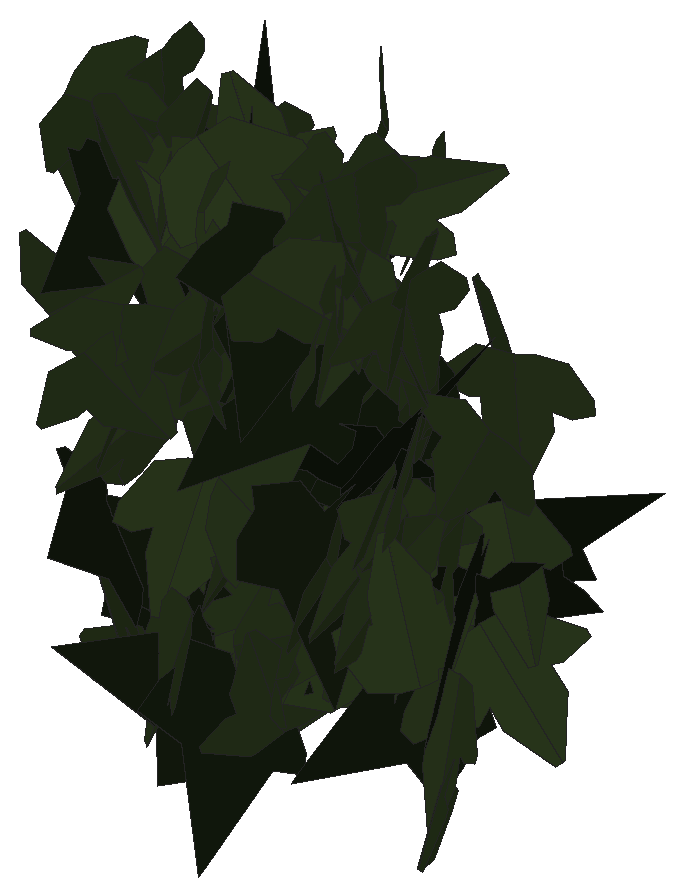
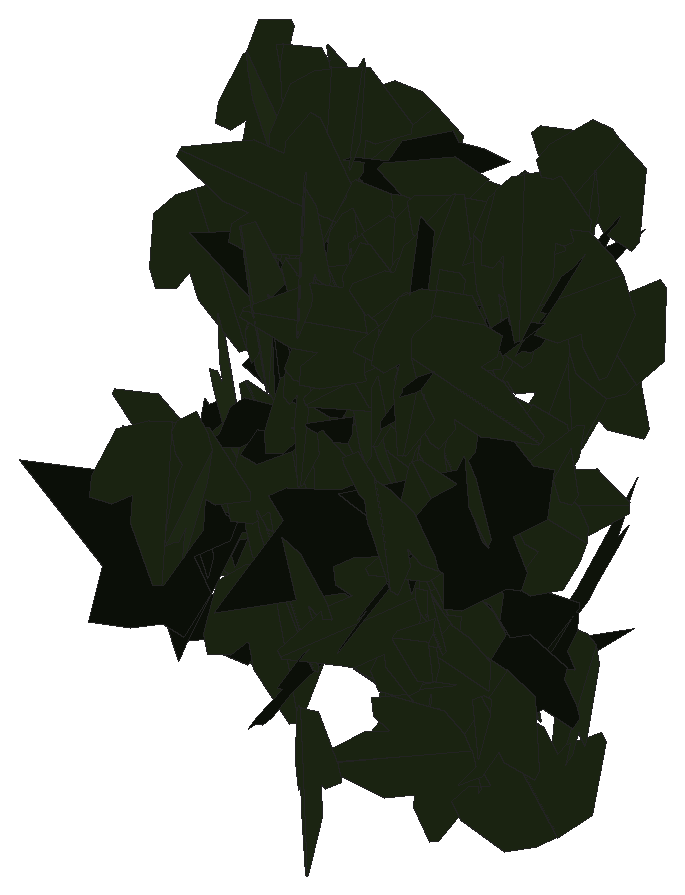
# SketchUp Ruby script. Lengths in inches.
U = 1.inch
M = Sketchup.active_model
def pt(a) = Geom::Point3d.new(a.map { |v| v * U })
def face(e, loops, mat)
  f = e.add_face(loops[0].map { |a| pt(a) })
  loops[1..].each { |l| e.add_face(l.map { |a| pt(a) }).erase! }
  f.material = f.back_material = mat if mat
  f
end
# faces: each face lists its corners as indices into pts; further lists are holes
def faces(e, pts, list, mat = nil) = list.each { |f| face(e, (f[0].is_a?(Array) ? f : [f]).map { |l| l.map { |i| pts[i] } }, mat) }
# xy, xz, yz: faces in a plane at the given z, y or x. An outline is a flat list of corners, or four numbers for a rectangle; further outlines are holes
def ring(l) = l.size == 4 ? [[l[0], l[1]], [l[2], l[1]], [l[2], l[3]], [l[0], l[3]]] : l.each_slice(2).to_a
def flat(e, list, mat, &to3) = list.each { |f| face(e, (f[0].is_a?(Array) ? f : [f]).map { |l| ring(l).map { |u, v| to3.(u, v) } }, mat) }
def xy(e, z, list, mat = nil) = flat(e, list, mat) { |x, y| [x, y, z] }
def xz(e, y, list, mat = nil) = flat(e, list, mat) { |x, z| [x, y, z] }
def yz(e, x, list, mat = nil) = flat(e, list, mat) { |y, z| [x, y, z] }
def lines(e, pts, list) = list.each { |a, b| e.add_line(pt(pts[a]), pt(pts[b])) }
# prism: a flat outline (further loops are holes) pulled along v
def prism(e, loops, v, mat = nil)
  f = face(e, loops, mat); d = Geom::Vector3d.new(v.map { |x| x * U })
  f.pushpull(f.normal.samedirection?(d) ? d.length : -d.length)
end
def box(e, o, s, mat = nil) = prism(e, [[o, [o[0] + s[0], o[1], o[2]], [o[0] + s[0], o[1] + s[1], o[2]], [o[0], o[1] + s[1], o[2]]]], [0, 0, s[2]], mat)
def at(x, y, z, deg = 0) = Geom::Transformation.translation(pt([x, y, z])) * Geom::Transformation.rotation(ORIGIN, Z_AXIS, deg.degrees)
def axes(o, x, y, z) = Geom::Transformation.new([*x, 0, *y, 0, *z, 0, *pt(o).to_a, 1])
def part(name) = M.definitions.add(name)
# library, detail: a bought-in or finely detailed component or shape, given as its bounding box
def library(name, o, s) = part(name).tap { |d| box(d.entities, o, s) }
def detail(e, o, s) = box(e.add_group.entities, o, s)
def put(e, d, t, mat = nil) = e.add_instance(d, t).tap { |i| i.material = mat if mat }
def group(e, t, mat = nil) = e.add_group.tap { |g| g.transformation = t; g.material = mat if mat }.entities
root = M.entities
M.materials.add("efeu1").color = [18, 25, 13]
M.materials.add("efeu2").color = [43, 57, 29]
c1 = part("ivyleaf_10")
p = [[0,0.5,-0.03],[-0.0625,2.02,-0.43],[-0.19,2.01,-0.46],[-0.54,1.05,-0.29],[-0.52,0.625,-0.18],[-0.83,0.76,-0.28],
  [-1.16,0.64,-0.33],[-1.15,0.33,-0.24],[-0.77,-0.39,0.02],[-0.3,-0.51,0.16],[0.04,-0.48,0.23],[-0.02,2.01,-0.4375],
  [-0.06,2.01,-0.43],[0.04,-0.49,0.23],[0.67,-0.49,0.14],[1.38,0.36,-0.2],[1.375,0.51,-0.24],[0.81,0.65,-0.19],
  [0.62,0.59,-0.15],[0.6,1.09,-0.28],[0.5,1.23,-0.31]]
faces(c1.entities,p,[[0,1,2,3,4,5,6,7,8,9,10],[11,12,0,13,14,15,16,17,18,19,20]],"efeu2")
c2 = part("ivyleaf_9")
p = [[1.54,2.16,1.25],[1.36,2.04,1.19],[-0.21,0.99,0.68],[-0.71,1.11,0.82],[-0.85,0.86,0.67],[-0.8,0.17,0.21],
  [-0.9,-0.01,0.1],[-0.67,-0.16,-0.02],[-0.08,-0.08,-0.05],[-0.03,-0.6,-0.4],[0.65,-0.88,-0.66],[0.83,-0.6,-0.49],
  [1.29,-0.42,-0.43],[1.8125,-0.07,-0.26],[1.21,0.44,0.15]]
faces(c2.entities,p,[[0,1,2,3,4,5,6,7,8,9,10,11,12,13,14]],"efeu1")
put(root,c1,axes([24.57,223.95,205.69],[-0.11682,0.10637,0.47438],[-0.34487,0.32575,-0.15797],[-0.34266,-0.36411,-0.00274]))
put(root,c1,axes([23.95,224.3125,202.88],[0.35736,-0.34773,-0.03714],[-0.02514,0.02743,-0.49861],[0.3488,0.35823,0.00212]))
put(root,c1,axes([25.12,224.07,206.5],[-0.27318,-0.1919,-0.37222],[0.30479,0.21365,-0.33385],[0.28718,-0.4093,0.00025]))
put(root,c1,axes([23.4375,224.29,205.45],[-0.40279,-0.29062,0.05747],[-0.04187,-0.04018,-0.49662],[0.29327,-0.40488,0.00803]))
put(root,c1,axes([22.87,224.29,205.4],[-0.33422,-0.06379,0.36637],[0.3582,0.07713,0.34021],[-0.09992,0.48988,-0.00586]))
put(root,c2,axes([24.93,224.52,206.46],[-0.27049,-0.41591,-0.06209],[0.03285,0.0527,-0.49613],[0.41924,-0.27247,-0.00118]))
put(root,c1,axes([24.61,224.3125,204.91],[-0.15567,-0.45543,0.13548],[0.0701,0.11899,0.48055],[-0.46995,0.16861,0.0268]))
put(root,c1,axes([26.24,224.26,206.63],[-0.18585,-0.43965,-0.14887],[0.05349,0.13901,-0.4773],[0.46108,-0.19334,-0.00464]))
put(root,c1,axes([24.77,224.08,204.48],[-0.00219,0.40153,0.29795],[-0.00192,0.29794,-0.40153],[-0.49999,-0.00291,0.00024]))
put(root,c2,axes([24.3125,224.65,202.32],[-0.11639,-0.48302,0.05608],[-0.01336,-0.05447,-0.49684],[0.48608,-0.11716,-0.00023]))
put(root,c1,axes([25.625,224.72,203.66],[-0.036,-0.03934,0.49715],[0.25855,-0.4277,-0.01512],[0.42645,0.25598,0.05114]))
put(root,c1,axes([23.3,224.2,205.09],[-0.28336,-0.30808,-0.27349],[0.17718,0.20853,-0.41848],[0.3719,-0.33407,-0.009]))
put(root,c1,axes([26.16,224.57,206.83],[0.22591,-0.4016,0.19412],[0.09855,-0.16728,-0.46077],[0.43503,0.24644,0.00357]))
put(root,c1,axes([25.63,224.75,204.15],[0.04581,-0.2235,0.44492],[0.10899,-0.43146,-0.22796],[0.48582,0.11787,0.00919]))
put(root,c2,axes([25.01,224.73,205.46],[-0.34584,-0.30956,0.18592],[-0.13083,-0.13252,-0.46403],[0.33657,-0.36961,0.01066]))
put(root,c2,axes([22.92,224.77,203.37],[0.28209,-0.27912,-0.30416],[0.21889,-0.21121,0.39684],[-0.35001,-0.35705,0.00303]))
put(root,c1,axes([25.25,224.63,206.56],[-0.15262,0.08956,0.46764],[0.41437,-0.2169,0.17678],[0.23452,0.44151,-0.00802]))
put(root,c1,axes([24.69,224.67,202.29],[-0.21464,-0.40409,-0.20159],[-0.08658,-0.18223,0.45749],[-0.44321,0.2313,0.00825]))
put(root,c2,axes([25.17,224.6,204.21],[-0.09776,-0.46401,-0.15855],[0.01898,0.15796,-0.47401],[0.48998,-0.0987,-0.01327]))
put(root,c1,axes([25.12,224.45,205.63],[0.27714,-0.41403,0.04202],[-0.01725,0.03901,0.49818],[-0.4158,-0.27758,0.00734]))
put(root,c1,axes([23.09,224.57,206.94],[-0.31088,0.21856,-0.32494],[0.25942,-0.19584,-0.37993],[-0.29334,-0.40482,0.00837]))
put(root,c2,axes([24.11,224.79,202.22],[-0.14487,-0.39163,-0.27502],[-0.0876,-0.26079,0.41751],[-0.47047,0.16915,0.00694]))
put(root,c1,axes([26.43,224.375,201.96],[0.27052,-0.35966,0.21786],[-0.13103,0.17405,0.45004],[-0.39956,-0.30058,-0.00009]))
put(root,c1,axes([24.4,224.87,204],[0.09608,-0.24805,0.42337],[0.1342,-0.40167,-0.2658],[0.47197,0.16471,-0.01061]))
put(root,c2,axes([23.03,224.95,206.03],[-0.10925,-0.28685,0.39469],[-0.09083,-0.38544,-0.30527],[0.47939,-0.1384,0.03211]))
put(root,c1,axes([26.33,224.68,202.94],[0.44053,-0.21342,0.10192],[0.09307,-0.04166,-0.48949],[0.21743,0.45024,0.00302]))
put(root,c1,axes([24.34,224.77,202.78],[0.1958,-0.1455,-0.43645],[0.33546,-0.27946,0.24366],[-0.31485,-0.38824,-0.01182]))
put(root,c1,axes([23.78,224.93,205.3],[-0.07333,0.08624,0.48702],[0.21879,-0.43589,0.11013],[0.44357,0.22926,0.0262]))
put(root,c1,axes([25.38,224.8,206.3],[0.01961,0.37311,-0.33227],[-0.03623,-0.33059,-0.37336],[-0.4983,0.03872,0.01407]))
put(root,c1,axes([25.32,224.45,203.92],[0.03509,-0.38631,-0.31549],[-0.01346,0.31542,-0.38772],[0.49859,0.0357,0.01173]))
put(root,c1,axes([23.12,225.03,204.28],[-0.01076,-0.14686,0.47782],[0.03165,-0.47718,-0.14595],[0.49888,0.02711,0.01957]))
put(root,c2,axes([25.77,224.34,204.92],[-0.07485,0.4794,-0.12073],[-0.03727,0.11628,0.48486],[0.49296,0.08159,0.01833]))
put(root,c1,axes([26,224.5625,205.76],[-0.29498,0.22202,-0.33719],[-0.2983,0.16153,0.36732],[0.27203,0.41787,0.03716]))
put(root,c1,axes([26.7,224.66,205.375],[-0.41664,-0.04093,0.27338],[-0.26963,-0.04881,-0.41823],[0.06093,-0.49593,0.0186]))
put(root,c1,axes([25.96,224.66,203.27],[0.16451,0.4717,0.02086],[-0.00695,-0.01967,0.49956],[0.47211,-0.16465,0.00008]))
put(root,c1,axes([25.77,224.78,204.51],[0.23603,-0.43595,-0.06509],[0.0358,-0.05463,0.49572],[-0.43933,-0.23867,0.00543]))
put(root,c1,axes([25.57,224.8,204.45],[0.25687,-0.42892,0.00667],[0.00341,-0.00573,-0.49996],[0.42896,0.25689,-0.00002]))
put(root,c1,axes([24.68,224.78,206.21],[0.48269,0.12391,0.04076],[0.03961,0.00966,-0.49834],[-0.12428,0.48431,-0.00049]))
put(root,c2,axes([25.87,225.16,202.75],[0.0077,-0.14569,-0.47824],[0.10224,-0.46773,0.14413],[-0.48938,-0.10001,0.02259]))
put(root,c1,axes([25.37,224.79,203.07],[0.34007,-0.01893,-0.36605],[-0.36326,0.04927,-0.34002],[0.04894,0.49721,0.01976]))
put(root,c1,axes([22.86,224.54,207.16],[-0.14634,-0.25614,-0.4037],[0.19156,0.35541,-0.29494],[0.43805,-0.24099,-0.00589]))
put(root,c1,axes([24.24,224.55,205.31],[0.06302,-0.28328,0.40716],[-0.05239,0.40434,0.28942],[-0.49324,-0.07914,0.02128]))
put(root,c1,axes([23.68,224.91,203.77],[0.39896,0.27519,-0.12287],[-0.10257,-0.06769,-0.48466],[-0.28339,0.41193,0.00244]))
put(root,c1,axes([24.48,224.83,203.03],[0.28595,-0.09191,-0.39973],[-0.3842,0.11058,-0.30026],[0.14361,0.47888,-0.00738]))
put(root,c1,axes([24.94,224.89,205.93],[-0.01665,-0.49692,-0.05283],[0.00196,0.0528,-0.4972],[0.49972,-0.01676,0.00019]))
put(root,c1,axes([25.26,224.86,207.02],[-0.19808,-0.45068,-0.08746],[0.03791,0.07887,-0.49228],[0.45752,-0.20165,0.00292]))
put(root,c1,axes([22.85,224.81,202.84],[-0.38887,0.31425,0.00542],[-0.00427,0.00333,-0.49997],[-0.31427,-0.38889,0.0001]))
put(root,c1,axes([24.7,224.99,205.85],[-0.33002,-0.15318,0.34297],[-0.31145,-0.1436,-0.36383],[0.20996,-0.45378,-0.00063]))
put(root,c2,axes([23.35,225.05,203.04],[-0.3022,-0.1329,-0.37551],[0.34915,0.13853,-0.33001],[0.19175,-0.46168,0.00908]))
put(root,c2,axes([23.57,224.87,202.96],[-0.38082,0.05971,0.31845],[0.29309,-0.146,0.37787],[0.13811,0.47447,0.07619]))
put(root,c1,axes([22.62,224.9375,206.39],[-0.2947,0.05452,-0.40022],[0.3946,-0.06698,-0.29968],[-0.08629,-0.49248,-0.00355]))
put(root,c1,axes([23.73,224.77,205.95],[-0.24072,-0.19796,-0.39098],[0.33642,0.20241,-0.30961],[0.28085,-0.41212,0.03575]))
put(root,c1,axes([25.14,225.03,203.39],[0.3323,-0.3727,-0.02585],[-0.01812,0.01848,-0.49933],[0.37316,0.3328,-0.00122]))
put(root,c1,axes([25.9,225.24,204.02],[0.14912,-0.26983,-0.39364],[0.20133,-0.33835,0.3082],[-0.4327,-0.25042,0.00774]))
put(root,c2,axes([25.07,224.78,204.78],[0.41607,0.25689,-0.10437],[-0.09364,-0.04697,-0.4889],[-0.26099,0.42638,0.00902]))
put(root,c1,axes([24.33,225.1875,202.79],[0.05318,-0.00388,0.49715],[0.46954,-0.16396,-0.0515],[0.16343,0.47234,-0.01379]))
put(root,c1,axes([23.34,224.85,206.39],[0.22943,0.19434,0.39949],[0.30941,0.25274,-0.30065],[-0.31879,0.38517,-0.00428]))
put(root,c1,axes([25.59,225.32,205.29],[-0.14901,0.07668,0.47108],[0.30105,-0.36785,0.1551],[0.37036,0.32986,0.06345]))
put(root,c1,axes([23.01,224.8,204],[0.14642,-0.33262,0.3434],[-0.11615,0.32363,0.363],[-0.46376,-0.18607,0.01751]))
put(root,c1,axes([25.37,225.04,203.56],[-0.39645,-0.12661,0.27713],[0.26796,0.07155,0.41602],[-0.145,0.47838,0.01112]))
put(root,c1,axes([23.85,224.91,206.72],[0.2915,0.27649,0.29763],[0.22432,0.19586,-0.40164],[-0.33869,0.36769,-0.00986]))
put(root,c1,axes([25.27,224.83,206.21],[-0.1457,0.39214,0.27386],[-0.11664,0.24851,-0.4179],[-0.46386,-0.18567,0.01906]))
put(root,c1,axes([24.26,225.09,202.52],[0.00786,0.00813,0.49987],[0.49133,0.09225,-0.00923],[-0.09237,0.49135,-0.00654]))
put(root,c1,axes([23.26,225.4,206.6875],[0.11913,-0.32441,0.36134],[0.19405,-0.30926,-0.34162],[0.44514,0.22163,0.05222]))
put(root,c1,axes([24.26,224.84,204.34],[-0.21552,0.30684,0.33075],[-0.18486,0.27431,-0.37494],[-0.41155,-0.28391,-0.00479]))
put(root,c2,axes([26.11,225.33,203.81],[-0.197,0.13527,-0.43919],[0.36551,-0.24353,-0.23896],[-0.27856,-0.41521,-0.00294]))
put(root,c1,axes([25.82,225.26,203.28],[-0.00087,0.04846,0.49765],[-0.42938,-0.25506,0.02408],[0.25619,-0.42731,0.04206]))
put(root,c1,axes([24.19,224.82,202.16],[-0.01064,-0.1761,-0.46784],[0.20827,0.42384,-0.16427],[0.45443,-0.19837,0.06433]))
put(root,c1,axes([23.33,225.02,204.85],[-0.27686,-0.31433,-0.27302],[0.21621,0.17166,-0.41688],[0.35581,-0.3489,0.04087]))
put(root,c1,axes([23.73,225.29,205.56],[0.36079,-0.11645,0.32599],[0.32387,-0.05272,-0.37727],[0.12224,0.48338,0.03739]))
put(root,c1,axes([25.17,225.57,203.79],[-0.04798,-0.04919,0.49526],[-0.18459,-0.4603,-0.0636],[0.46219,-0.18895,0.02601]))
put(root,c1,axes([23.73,225.03,203.28],[0.2605,0.11677,-0.4105],[0.32199,0.26187,0.27883],[0.28011,-0.40962,0.06124]))
put(root,c1,axes([25.47,225.32,202.83],[-0.41262,-0.25051,0.13035],[-0.11277,-0.06542,-0.4827],[0.2589,-0.42774,-0.00251]))
put(root,c1,axes([22.88,225.28,201.85],[-0.23892,-0.4018,0.1774],[0.10237,0.14544,0.4673],[-0.42713,0.25961,0.01277]))
put(root,c1,axes([25.61,225.35,204.09],[-0.41766,-0.11924,0.24768],[-0.22597,-0.10759,-0.43285],[0.15652,-0.4735,0.03598]))
put(root,c1,axes([23.93,224.96,206.29],[0.00006,0.17514,0.46832],[-0.0177,0.46803,-0.17503],[-0.49969,-0.01656,0.00626]))
put(root,c2,axes([23.91,225.1,205.41],[0.12134,0.0028,0.48505],[0.4635,0.14673,-0.11679],[-0.14299,0.47798,0.03301]))
put(root,c1,axes([22.97,225.32,207.1],[-0.05884,-0.48145,-0.12141],[0.0248,0.11926,-0.48493],[0.49591,-0.06309,0.00985]))
put(root,c2,axes([25.18,225.68,204.2],[-0.34178,-0.16161,0.32721],[-0.28388,-0.16399,-0.37752],[0.22934,-0.44383,0.02034]))
put(root,c1,axes([24.37,225.49,205.16],[0.1536,-0.46831,0.08423],[0.03572,-0.07691,-0.49276],[0.47448,0.15739,0.00983]))
put(root,c1,axes([24.42,225.38,204.65],[0.21249,-0.03534,-0.45122],[-0.44123,0.09488,-0.21521],[0.10083,0.48964,0.00913]))
put(root,c1,axes([23.625,225.34,203.4],[0.26723,0.10696,0.40884],[0.371,0.17224,-0.28756],[-0.20235,0.45705,0.01269]))
put(root,c1,axes([26.31,225.29,203.12],[0.25946,0.3489,0.24689],[0.14993,0.19617,-0.43479],[-0.40025,0.29965,-0.00283]))
put(root,c1,axes([26.2,225.52,204.03],[0.43662,0.02997,0.24179],[0.24147,0.01292,-0.43764],[-0.03248,0.49893,-0.00319]))
put(root,c1,axes([24.19,225.41,203.89],[0.29571,-0.24751,-0.31827],[-0.25083,0.19607,-0.38554],[0.31565,0.38768,-0.00821]))
put(root,c1,axes([24.82,225.49,204.91],[-0.19714,-0.45873,-0.02662],[0.01455,0.02272,-0.49927],[0.45927,-0.19762,0.00439]))
put(root,c1,axes([23.29,225.4,202.37],[-0.2006,-0.04432,-0.45585],[0.4531,0.0534,-0.20458],[0.06682,-0.49516,0.01874]))
put(root,c1,axes([23.625,225.13,202.92],[0.06971,0.2094,-0.44866],[0.14188,0.42563,0.2207],[0.47435,-0.15808,-0.00008]))
put(root,c1,axes([23.92,225.52,205.91],[-0.20071,-0.03001,0.45696],[-0.44736,-0.09382,-0.20266],[0.0979,-0.4902,0.01081]))
put(root,c2,axes([26.21,225.36,203.6875],[0.26567,0.37857,-0.19],[-0.11573,-0.15087,-0.46243],[-0.40746,0.28969,0.00746]))
put(root,c2,axes([25.27,225.64,204.36],[-0.34086,-0.348,-0.11273],[-0.06017,-0.09865,0.48646],[-0.36082,0.3452,0.02538]))
put(root,c1,axes([24.56,225.58,205.95],[0.48501,0.01356,-0.12076],[-0.12066,-0.00532,-0.48519],[-0.01444,0.49979,-0.00188]))
put(root,c1,axes([23.25,225.47,202.78],[-0.4557,-0.03828,-0.20218],[0.20168,0.01442,-0.45729],[0.04084,-0.49832,0.0023]))
put(root,c1,axes([23.89,225.46,204.09],[0.34895,0.32023,0.16027],[0.11507,0.11164,-0.4736],[-0.33911,0.36741,0.00422]))
put(root,c1,axes([23.61,225.55,203.21],[0.38852,0.04189,0.31193],[0.30702,0.05859,-0.39027],[-0.06925,0.49479,0.0198]))
put(root,c1,axes([24.89,225.47,205.23],[0.01946,-0.44857,-0.22001],[0.01317,0.22056,-0.44853],[0.49945,0.01166,0.0204]))
put(root,c1,axes([24.76,225.46,205.45],[0.14618,-0.4133,0.24044],[-0.08529,0.22485,0.43837],[-0.47049,-0.16918,-0.00476]))
put(root,c1,axes([23.77,225.62,206.16],[0.21429,0.44537,0.07568],[-0.03823,-0.06559,0.4942],[0.45013,-0.21759,0.00594]))
put(root,c1,axes([23.875,225.59,203.125],[0.00639,-0.04048,0.49832],[0.47932,0.14221,0.0054],[-0.14217,0.47764,0.04062]))
put(root,c2,axes([24.73,226.0625,202.62],[-0.13506,-0.29466,0.3807],[-0.06906,-0.37945,-0.31819],[0.47643,-0.13853,0.0618]))
put(root,c1,axes([25.01,225.53,206.51],[-0.15025,-0.16764,0.44645],[0.31954,0.31208,0.22473],[-0.35401,0.35285,0.01335]))
put(root,c1,axes([23.88,225.43,205.625],[-0.11398,-0.12336,-0.47095],[0.31465,0.35042,-0.16794],[0.37149,-0.33465,-0.00225]))
put(root,c2,axes([23.78,225.58,206.01],[-0.01022,-0.26555,0.42353],[0.08527,0.41648,0.26319],[-0.49257,0.07761,0.03678]))
put(root,c2,axes([23.18,226.01,205.93],[-0.06057,-0.49545,0.02925],[0.00038,-0.02952,-0.49913],[0.49632,-0.06044,0.00395]))
put(root,c1,axes([24.96,225.74,204.33],[-0.45474,-0.10478,0.17953],[-0.17438,-0.04275,-0.46665],[0.11315,-0.48702,0.00234]))
put(root,c1,axes([23.77,225.55,205.875],[0.01284,0.45005,0.21747],[-0.01192,0.21776,-0.44993],[-0.49969,0.00637,0.01632]))
put(root,c1,axes([23.53,225.71,202.27],[-0.14962,-0.04741,-0.47473],[0.47611,0.01711,-0.15176],[0.03064,-0.49745,0.04002]))
put(root,c1,axes([23.4,225.55,204.91],[0.08598,0.39356,-0.29618],[0.05691,0.29071,0.4028],[0.48925,-0.10298,0.00519]))
put(root,c1,axes([23.875,225.69,203.47],[-0.16754,-0.11363,-0.45719],[0.37724,0.25829,-0.20243],[0.28218,-0.41277,-0.00082]))
put(root,c1,axes([23.85,226,205.71],[0.29667,-0.0077,0.4024],[0.40245,-0.00018,-0.29671],[0.00471,0.49994,0.0061]))
put(root,c1,axes([23.34,225.77,205],[0.09798,-0.10341,-0.47928],[-0.32176,0.35523,-0.14242],[0.36996,0.33633,0.00306]))
put(root,c1,axes([24.77,226.07,203.75],[0.43766,-0.2402,-0.0275],[-0.02423,0.01302,-0.49924],[0.24055,0.43833,-0.00024]))
put(root,c2,axes([24.12,225.89,204.12],[0.02763,-0.13563,-0.48046],[0.21217,0.43877,-0.11166],[0.45191,-0.19771,0.0818]))
put(root,c2,axes([23.4,226.08,204.33],[0.26201,-0.39955,-0.14733],[-0.05769,0.13809,-0.47708],[0.42193,0.267,0.02626]))
put(root,c1,axes([23.36,225.99,206.24],[-0.1526,-0.43851,-0.18552],[0.05907,0.17588,-0.4643],[0.47247,-0.16363,-0.00187]))
put(root,c1,axes([23.2,225.9,204.33],[0.29553,0.34254,-0.21291],[0.1157,0.18085,0.45156],[0.38636,-0.31616,0.02763]))
put(root,c2,axes([22.55,226.1,204.73],[0.29723,-0.10446,0.38826],[0.37771,-0.09295,-0.31416],[0.13781,0.48005,0.02365]))
put(root,c1,axes([23.2,226.15,205.99],[0.18813,0.02013,-0.46282],[-0.45985,0.06855,-0.18394],[0.05605,0.49487,0.04431]))
put(root,c1,axes([24.01,225.97,205.9375],[-0.08136,-0.14576,0.47131],[0.20814,0.42294,0.16673],[-0.44728,0.22333,-0.00815]))
put(root,c1,axes([24.95,226.22,206.36],[0.19211,-0.4193,-0.19308],[-0.08544,0.17322,-0.46119],[0.45365,0.21019,-0.0051]))
put(root,c1,axes([24.49,226.1,206.84],[0.1084,-0.2734,-0.40435],[-0.12682,0.38421,-0.29377],[0.47135,0.16625,0.01395]))
put(root,c2,axes([25.63,226.17,203.51],[0.30438,0.31505,-0.24102],[0.13741,0.20125,0.4366],[0.37211,-0.33202,0.03593]))
put(root,c1,axes([24.26,226.4,202.4375],[0.138,-0.40262,-0.2624],[-0.07522,0.25154,-0.42552],[0.47465,0.15692,0.00885]))
put(root,c1,axes([25.42,226.68,204.66],[-0.46326,-0.18581,0.02943],[-0.02704,-0.01163,-0.49913],[0.18617,-0.46405,0.00073]))
put(root,c1,axes([23.08,226.93,205.21],[0.46145,-0.1404,0.13172],[0.12455,-0.04313,-0.48231],[0.1468,0.47794,-0.00483]))
put(root,c1,axes([24.87,227,204.9],[-0.29862,0.34675,-0.20147],[0.1305,-0.1535,-0.45761],[-0.37921,-0.32588,0.00118]))
